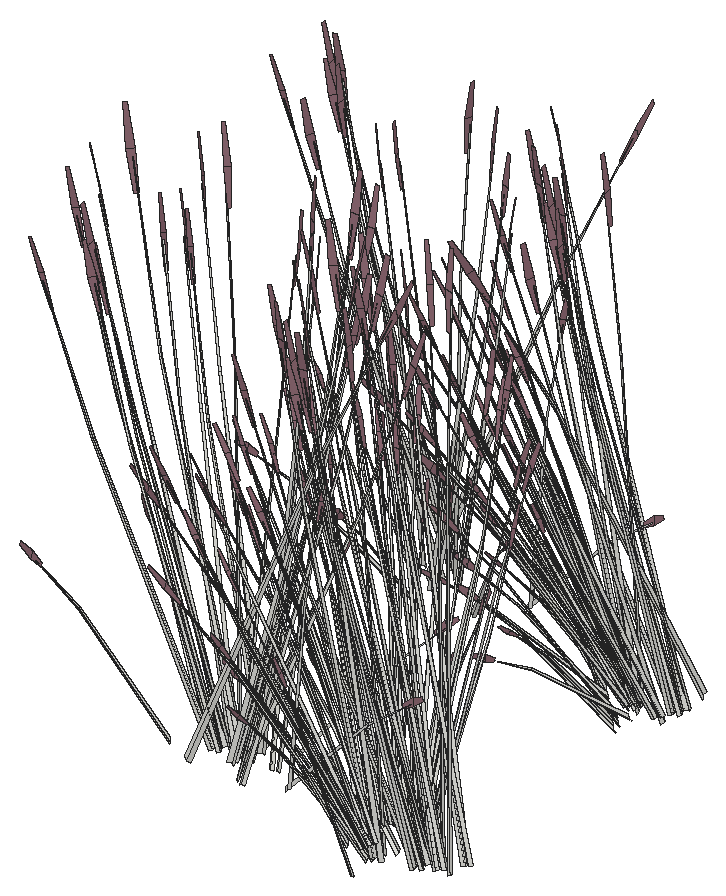
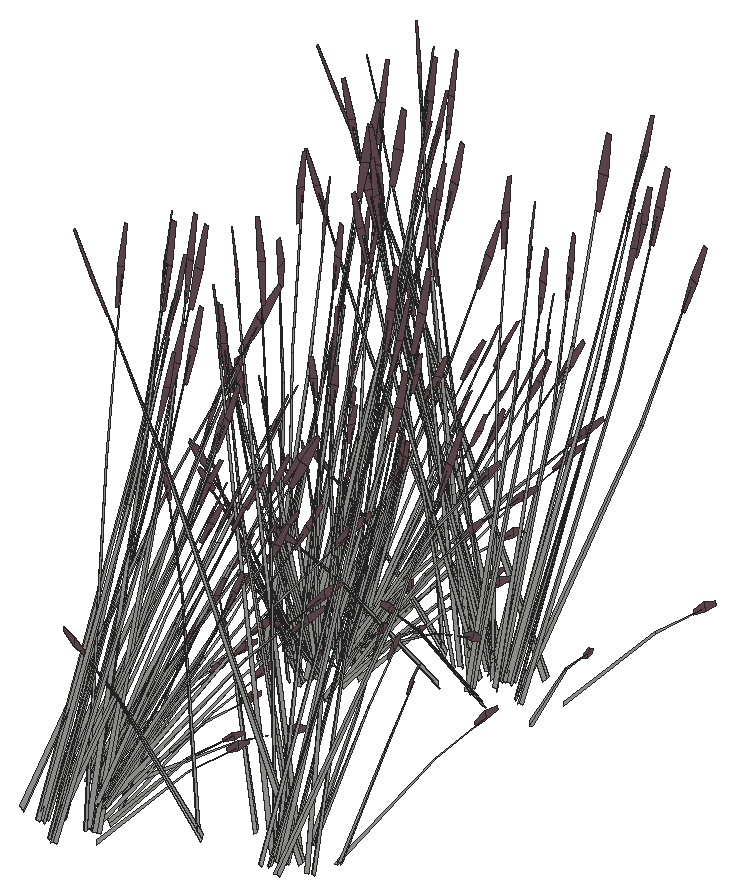
# SketchUp Ruby script. Lengths in inches.
U = 1.inch
M = Sketchup.active_model
def pt(a) = Geom::Point3d.new(a.map { |v| v * U })
def face(e, loops, mat)
  f = e.add_face(loops[0].map { |a| pt(a) })
  loops[1..].each { |l| e.add_face(l.map { |a| pt(a) }).erase! }
  f.material = f.back_material = mat if mat
  f
end
# faces: each face lists its corners as indices into pts; further lists are holes
def faces(e, pts, list, mat = nil) = list.each { |f| face(e, (f[0].is_a?(Array) ? f : [f]).map { |l| l.map { |i| pts[i] } }, mat) }
# xy, xz, yz: faces in a plane at the given z, y or x. An outline is a flat list of corners, or four numbers for a rectangle; further outlines are holes
def ring(l) = l.size == 4 ? [[l[0], l[1]], [l[2], l[1]], [l[2], l[3]], [l[0], l[3]]] : l.each_slice(2).to_a
def flat(e, list, mat, &to3) = list.each { |f| face(e, (f[0].is_a?(Array) ? f : [f]).map { |l| ring(l).map { |u, v| to3.(u, v) } }, mat) }
def xy(e, z, list, mat = nil) = flat(e, list, mat) { |x, y| [x, y, z] }
def xz(e, y, list, mat = nil) = flat(e, list, mat) { |x, z| [x, y, z] }
def yz(e, x, list, mat = nil) = flat(e, list, mat) { |y, z| [x, y, z] }
def lines(e, pts, list) = list.each { |a, b| e.add_line(pt(pts[a]), pt(pts[b])) }
# prism: a flat outline (further loops are holes) pulled along v
def prism(e, loops, v, mat = nil)
  f = face(e, loops, mat); d = Geom::Vector3d.new(v.map { |x| x * U })
  f.pushpull(f.normal.samedirection?(d) ? d.length : -d.length)
end
def box(e, o, s, mat = nil) = prism(e, [[o, [o[0] + s[0], o[1], o[2]], [o[0] + s[0], o[1] + s[1], o[2]], [o[0], o[1] + s[1], o[2]]]], [0, 0, s[2]], mat)
def at(x, y, z, deg = 0) = Geom::Transformation.translation(pt([x, y, z])) * Geom::Transformation.rotation(ORIGIN, Z_AXIS, deg.degrees)
def axes(o, x, y, z) = Geom::Transformation.new([*x, 0, *y, 0, *z, 0, *pt(o).to_a, 1])
def part(name) = M.definitions.add(name)
# library, detail: a bought-in or finely detailed component or shape, given as its bounding box
def library(name, o, s) = part(name).tap { |d| box(d.entities, o, s) }
def detail(e, o, s) = box(e.add_group.entities, o, s)
def put(e, d, t, mat = nil) = e.add_instance(d, t).tap { |i| i.material = mat if mat }
def group(e, t, mat = nil) = e.add_group.tap { |g| g.transformation = t; g.material = mat if mat }.entities
root = M.entities
M.materials.add("LightPink_Translucent").color = [144, 107, 117]
c1 = part("blade")
p = [[2.15,0.21,22],[0,0.17,0],[0.09,0.45,0],[2.18,0.31,22],[2.29,0.31,22],[0.38,0.45,0],
  [2.48,0.24,33],[2.49,0.24,33],[2.48,0.22,33]]
faces(c1.entities,p,[[0,1,2,3],[4,5,2,3],[6,3,4,7],[8,0,3,6]])
c2 = part("seeds")
p = [[0.3,-0.1,1.38],[-0.01,-0.03,1.59],[-0.01,-0.03,0.03],[0.14,-0.07,-0.07],[0.29,-0.03,3],[0.15,0.01,3.11]]
faces(c2.entities,p,[[0,1,2,3],[1,0,4,5]],"LightPink_Translucent")
c3 = part("blade with seeds")
put(c3.entities,c1,at(0,0,0))
put(c3.entities,c2,axes([2.4,0.25,30.99],[1.5799,-0.05474,1.17369],[-0.12525,1.92788,0.29478],[-0.07173,-0.02425,1.56792]))
put(root,c3,axes([47.72,595.87,44.06],[-1.27479,-0.1698,-0.62353],[0.26901,-1.04736,-0.16365],[-0.38043,-0.12691,1.37633]))
put(root,c3,axes([47.45,555.5625,43.49],[0.03108,0.16322,1.76342],[-0.62654,0.85237,-0.26939],[-0.44504,-0.04296,0.30037]))
put(root,c3,axes([45.54,590.14,43.49],[-0.11871,0.13643,1.76342],[-1.19964,0.29415,-0.26939],[-0.2898,-0.26759,0.30037]))
put(root,c3,axes([47.12,560.13,43.49],[0.16438,0.10347,1.76342],[0.27873,0.95868,-0.26939],[-0.36432,0.20444,0.30037]))
put(root,c3,axes([44.8,590.66,44.13],[-0.35352,0.84566,-0.03893],[-1.08806,-0.26014,-0.17649],[-0.1652,-0.13832,0.58215]))
put(root,c3,axes([51.55,557.04,44.06],[-1.27479,-0.1698,-0.62353],[0.26901,-1.04736,-0.16365],[-0.38043,-0.12691,1.37633]))
put(root,c3,axes([48.38,595.54,44.21],[-0.73619,-0.86927,-0.44739],[1.11511,-0.61213,0.21531],[-0.23824,-0.10756,1.43643]))
put(root,c3,axes([49.88,559.03,44.02],[-1.14694,-0.51783,-0.49651],[0.68554,-0.92854,0],[-0.26122,-0.11794,1.57504]))
put(root,c3,axes([48.49,596.03,44.4375],[0.32481,-1.2272,-0.23429],[1.54007,0.21392,0.51271],[-0.26911,-0.16947,1.5644]))
put(root,c3,axes([44.56,593.74,44.02],[0,-1.03566,-0.49651],[1.37109,0,0],[0,-0.23588,1.57504]))
put(root,c3,axes([48.14,594.9375,44.67],[-1.38012,-0.49416,-0.29095],[0.66454,-1.04299,-0.50002],[-0.04337,-0.25608,1.59708]))
put(root,c3,axes([53,557.2,44.67],[-1.23732,0.68758,-0.29095],[-0.8228,-0.97154,-0.50002],[-0.30528,-0.09867,1.59708]))
put(root,c3,axes([50.2,558.64,44.03],[-0.28787,-0.90242,-0.30978],[1.14332,-0.25625,0.30978],[-0.23049,-0.10406,1.38974]))
put(root,c3,axes([47.52,593.89,44.1],[-0.50328,-1.06202,-0.69835],[1.44974,-0.38248,-0.18329],[-0.05563,-0.35963,1.54149]))
put(root,c3,axes([53.82,557.95,44.06],[-0.82544,0.77843,-0.62353],[-1.0254,-0.70586,-0.16365],[-0.33076,0.19418,1.37633]))
put(root,c3,axes([45.15,593.76,44.03],[0.85545,-0.64616,-0.30978],[0.85545,0.64616,0.30978],[0,-0.20813,1.38974]))
put(root,c3,axes([49.01,589.58,44.13],[-0.84686,0.59414,-0.03893],[-0.77596,-0.65071,-0.17649],[-0.05463,-0.18438,0.58215]))
put(root,c3,axes([54.39,557.51,44.46],[-1.19666,-0.83357,-0.25192],[1.00694,-0.93603,0.5513],[-0.32224,0.09751,1.68216]))
put(root,c3,axes([52.21,556.71,44.21],[-0.73619,-0.86927,-0.44739],[1.11511,-0.61213,0.21531],[-0.23824,-0.10756,1.43643]))
put(root,c3,axes([53.78,557.33,44.21],[-1.33077,0.06393,-0.44739],[-0.12035,-1.06125,0.21531],[-0.23824,0.10756,1.43643]))
put(root,c3,axes([52.32,557.21,44.4375],[0.32481,-1.2272,-0.23429],[1.54007,0.21392,0.51271],[-0.26911,-0.16947,1.5644]))
put(root,c3,axes([55.18,560.07,44.02],[-1.14694,0.51783,-0.49651],[-0.68554,-0.92854,0],[-0.26122,0.11794,1.57504]))
put(root,c3,axes([49.22,588.86,43.49],[-0.20555,0.03731,1.76342],[-1.13672,-0.42002,-0.26939],[0.01907,-0.35034,0.30037]))
put(root,c3,axes([54.91,559.66,44.03],[-1.14332,-0.25625,-0.30978],[0.28787,-0.90242,0.30978],[-0.23049,0.10406,1.38974]))
put(root,c3,axes([48.29,594.16,44.21],[0.59459,-0.93321,-0.44739],[1.23546,0.44912,0.21531],[0,-0.21512,1.43643]))
put(root,c3,axes([54.71,557.05,44.67],[0.1428,1.18174,-0.29095],[-1.48733,0.07145,-0.50002],[-0.26191,0.15741,1.59708]))
put(root,c3,axes([52.19,560.23,43.49],[0.19833,-0.05635,1.76342],[1.19302,0.31018,-0.26939],[0.03489,0.3496,0.30037]))
put(root,c3,axes([48.83,593.7,44.67],[-0.1428,-1.18174,-0.29095],[1.48733,-0.07145,-0.50002],[0.26191,-0.15741,1.59708]))
put(root,c3,axes([55.26,556.58,44.21],[-0.59459,0.93321,-0.44739],[-1.23546,-0.44912,0.21531],[0,0.21512,1.43643]))
put(root,c3,axes([48.64,591.08,44.03],[1.14332,0.25625,-0.30978],[-0.28787,0.90242,0.30978],[0.23049,-0.10406,1.38974]))
put(root,c3,axes([48.37,590.67,44.02],[1.14694,-0.51783,-0.49651],[0.68554,0.92854,0],[0.26122,-0.11794,1.57504]))
put(root,c3,axes([58.4,556.98,44.03],[-0.85545,0.64616,-0.30978],[-0.85545,-0.64616,0.30978],[0,0.20813,1.38974]))
put(root,c3,axes([49.73,592.8,44.06],[0.82544,-0.77843,-0.62353],[1.0254,0.70586,-0.16365],[0.33076,-0.19418,1.37633]))
put(root,c3,axes([55.96,556.87,44.09],[0.44936,0.94823,-0.69212],[-1.29441,0.3415,-0.18165],[0.04967,0.32109,1.52773]))
put(root,c3,axes([69.75,555.49,41.15],[0.50831,-0.02346,1.71376],[-0.33721,1.01661,0.13857],[-0.72439,-0.06288,0.73262]))
put(root,c3,axes([69.75,591.94,40.8125],[0.50831,-0.02346,1.71376],[-0.33721,1.01661,0.13857],[-0.72439,-0.06288,0.73262]))
put(root,c3,axes([55.4,555.81,44.67],[1.38012,0.49416,-0.29095],[-0.66454,1.04299,-0.50002],[0.04337,0.25608,1.59708]))
put(root,c3,axes([69.96,557.28,41.15],[0.42521,-0.21906,1.71376],[0.35798,1.01226,0.13857],[-0.66754,0.22878,0.73262]))
put(root,c3,axes([58.99,557.01,44.02],[0,1.03566,-0.49651],[-1.37109,0,0],[0,0.23588,1.57504]))
put(root,c3,axes([68.64,559,39.87],[0.42589,0.08502,1.43002],[0.2745,0.86839,-0.30754],[-0.57851,0.16255,0.61141]))
put(root,c3,axes([47.43,592.93,43.59],[-1.20625,0.41464,1.28929],[-0.38394,-1.1897,0.50096],[0.74071,0.01979,1.46642]))
put(root,c3,axes([72.41,556.22,40.62],[0.34834,-0.14982,1.77064],[0.12012,1.04605,0.13857],[-0.75452,0.1388,0.63284]))
put(root,c3,axes([54.25,590.64,43.49],[-0.18342,-0.08159,1.76342],[-0.47115,-0.9115,-0.26939],[0.31784,-0.24736,0.30037]))
put(root,c3,axes([55.14,558.22,44.18],[1.2866,-0.3514,-0.19198],[0.45209,1.01223,0.00008],[0.14202,-0.03884,1.73897]))
put(root,c3,axes([68.66,556.92,41.99],[-0.20012,0.13446,1.74944],[0.01702,0.98243,-0.27667],[-0.45871,0.12776,0.14031]))
put(root,c3,axes([71.27,554.54,42.26],[-1.22504,-0.02494,-0.71045],[0.08228,-1.05005,0.08574],[-0.51899,-0.11081,1.00501]))
put(root,c3,axes([71.27,590.99,41.92],[-1.22504,-0.02494,-0.71045],[0.08228,-1.05005,0.08574],[-0.51899,-0.11081,1.00501]))
put(root,c3,axes([70.29,554.8,39.87],[0.23927,0.28834,1.43002],[-0.55135,0.78376,-0.30754],[-0.56612,-0.18733,0.61141]))
put(root,c3,axes([70.29,591.25,39.53],[0.23927,0.28834,1.43002],[-0.55135,0.78376,-0.30754],[-0.56612,-0.18733,0.61141]))
put(root,c3,axes([55.16,555.21,44.21],[0.73619,0.86927,-0.44739],[-1.11511,0.61213,0.21531],[0.23824,0.10756,1.43643]))
put(root,c3,axes([69.31,556.36,41.8],[-1.01846,-0.28891,-0.35414],[0.29705,-0.84289,0.4572],[-0.41005,0.07729,0.87481]))
put(root,c3,axes([69.31,592.81,41.46],[-1.01846,-0.28891,-0.35414],[0.29705,-0.84289,0.4572],[-0.41005,0.07729,0.87481]))
put(root,c3,axes([70.71,590.3,40.8125],[0.45521,0.17844,1.71376],[-0.94204,0.74856,0.13857],[-0.58713,-0.33769,0.73262]))
put(root,c3,axes([57.42,594.32,44.26],[-0.75977,-0.66224,-0.06488],[0.83212,-0.6068,-0.29416],[0.23578,-0.04272,0.97024]))
put(root,c3,axes([66.4375,557.91,41.99],[0.1564,0.02778,1.77383],[0.48382,0.91506,-0.16761],[-0.32016,0.24017,0.31391]))
put(root,c3,axes([70,556.79,41.96],[-0.332,0.94205,-0.51099],[-1.13828,-0.3229,-0.3958],[-0.45829,0.08638,0.97773]))
put(root,c3,axes([70.87,554.75,41.96],[-0.88986,0.68603,-0.51099],[-0.77932,-0.72471,-0.3958],[-0.45212,-0.10438,0.97773]))
put(root,c3,axes([70.87,591.2,41.62],[-0.88986,0.68603,-0.51099],[-0.77932,-0.72471,-0.3958],[-0.45212,-0.10438,0.97773]))
put(root,c3,axes([69.43,556.73,38.77],[0.03108,0.16322,1.76342],[-0.62654,0.85237,-0.26939],[-0.44504,-0.04296,0.30037]))
put(root,c3,axes([69.43,593.18,38.43],[0.03108,0.16322,1.76342],[-0.62654,0.85237,-0.26939],[-0.44504,-0.04296,0.30037]))
put(root,c3,axes([57.18,553.28,44.03],[0.28787,0.90242,-0.30978],[-1.14332,0.25625,0.30978],[0.23049,0.10406,1.38974]))
put(root,c3,axes([69.61,552.83,41.99],[0.09085,0.10335,1.77383],[-0.43798,0.92907,-0.16761],[-0.44357,0.00672,0.31391]))
put(root,c3,axes([69.61,589.28,41.64],[0.09085,0.10335,1.77383],[-0.43798,0.92907,-0.16761],[-0.44357,0.00672,0.31391]))
put(root,c3,axes([67.75,560.82,40.04],[0.51072,-0.46938,1.1486],[0.20153,0.74307,0.84392],[-0.36908,0.13305,0.25299]))
put(root,c3,axes([54.38,554.72,44.67],[1.23732,-0.68758,-0.29095],[0.8228,0.97154,-0.50002],[0.30528,0.09867,1.59708]))
put(root,c3,axes([70.625,588.66,41.65],[-0.26368,-0.00731,1.74944],[-0.83946,0.73103,-0.27667],[-0.44791,-0.14937,0.14031]))
put(root,c3,axes([69.54,556.26,42.01],[0.34623,-0.9443,0.48003],[1.13828,0.3229,0.3958],[-0.44763,0.05675,0.9933]))
put(root,c3,axes([69.54,592.7,41.67],[0.34623,-0.9443,0.48003],[1.13828,0.3229,0.3958],[-0.44763,0.05675,0.9933]))
put(root,c3,axes([69.95,555.98,42.3125],[0.6166,0.93779,-0.1216],[-1.09436,0.46085,-0.67495],[-0.46117,0.12373,1.02557]))
put(root,c3,axes([71.33,554.04,42.3125],[-0.06562,1.05324,-0.1216],[-1.2424,-0.02879,-0.67495],[-0.4785,-0.07316,1.02557]))
put(root,c3,axes([71.33,590.48,41.97],[-0.06562,1.05324,-0.1216],[-1.2424,-0.02879,-0.67495],[-0.4785,-0.07316,1.02557]))
put(root,c3,axes([70.54,554.11,41.8],[-0.69728,-0.64842,-0.35414],[0.79619,-0.61382,0.4572],[-0.40453,-0.09339,0.87481]))
put(root,c3,axes([70.54,590.56,41.46],[-0.69728,-0.64842,-0.35414],[0.79619,-0.61382,0.4572],[-0.40453,-0.09339,0.87481]))
put(root,c3,axes([69.46,556,42.01],[-0.4501,-0.70615,0.0643],[0.82077,-0.34564,0.50621],[-0.36181,0.0682,0.77189]))
put(root,c3,axes([69.46,592.45,41.67],[-0.4501,-0.70615,0.0643],[0.82077,-0.34564,0.50621],[-0.36181,0.0682,0.77189]))
put(root,c3,axes([71.52,557.96,41.15],[0.30609,-0.31822,1.71376],[0.77286,0.85893,0.13857],[-0.53009,0.39116,0.73262]))
put(root,c3,axes([69.68,558.79,41.8],[-1.06674,0.14801,-0.35414],[-0.28168,-0.84611,0.4572],[-0.30569,0.22726,0.87481]))
put(root,c3,axes([69.1,561.3,38.77],[0.16438,0.10347,1.76342],[0.27873,0.95868,-0.26939],[-0.36432,0.20444,0.30037]))
put(root,c3,axes([51.26,554.11,43.59],[-1.20625,0.41464,1.28929],[-0.38394,-1.1897,0.50096],[0.74071,0.01979,1.46642]))
put(root,c3,axes([68.86,555.66,40.04],[0.78239,-0.07411,1.1486],[-0.49629,0.65296,0.84392],[-0.38663,-0.09795,0.25299]))
put(root,c3,axes([68.86,592.11,39.7],[0.78239,-0.07411,1.1486],[-0.49629,0.65296,0.84392],[-0.38663,-0.09795,0.25299]))
put(root,c3,axes([69.82,558.61,42.01],[-0.30393,-0.95317,0.48003],[1.19224,-0.16542,0.3958],[-0.35138,0.22417,0.9933]))
put(root,c3,axes([70.43,590.3125,42.03],[1.01205,-0.7643,0.53763],[0.87284,0.81167,0.4433],[-0.47482,-0.14098,1.11249]))
put(root,c3,axes([69.58,558.42,42.01],[-0.8413,-0.43556,0.0643],[0.48981,-0.62025,0.50621],[-0.26973,0.20053,0.77189]))
put(root,c3,axes([57.5,552.89,44.02],[1.14694,0.51783,-0.49651],[-0.68554,0.92854,0],[0.26122,0.11794,1.57504]))
put(root,c3,axes([57.44,560.26,43.49],[0.08928,-0.14952,1.76342],[1.12407,-0.44035,-0.26939],[0.34078,0.22791,0.30037]))
put(root,c3,axes([71.29,558.74,41.15],[0.22818,-0.35597,1.71376],[0.95725,0.73667,0.13857],[-0.43183,0.45914,0.73262]))
put(root,c3,axes([70.38,556.27,42.33],[1.01846,0.28891,0.35414],[-0.29705,0.84289,-0.4572],[-0.41005,0.07729,0.87481]))
put(root,c3,axes([55.83,554.875,44.06],[1.27479,0.1698,-0.62353],[-0.26901,1.04736,-0.16365],[0.38043,0.12691,1.37633]))
put(root,c3,axes([70.56,558.89,41.96],[0.31482,0.94565,-0.51099],[-1.19224,0.16542,-0.3958],[-0.34166,0.254,0.97773]))
put(root,c3,axes([61.25,555.49,44.26],[-0.75977,-0.66224,-0.06488],[0.83212,-0.6068,-0.29416],[0.23578,-0.04272,0.97024]))
put(root,c3,axes([70.89,553.86,42.01],[0.06171,-0.78753,0.0643],[0.9318,0.02159,0.50621],[-0.35694,-0.08241,0.77189]))
put(root,c3,axes([70.89,590.31,41.67],[0.06171,-0.78753,0.0643],[0.9318,0.02159,0.50621],[-0.35694,-0.08241,0.77189]))
put(root,c3,axes([68.7,560.59,41.99],[-0.03046,0.20495,1.74944],[0.86449,0.71297,-0.27667],[-0.22632,0.33716,0.14031]))
put(root,c3,axes([73.53,558.21,39.34],[-1.27479,-0.1698,-0.62353],[0.26901,-1.04736,-0.16365],[-0.38043,-0.12691,1.37633]))
put(root,c3,axes([73.53,594.66,38.99],[-1.27479,-0.1698,-0.62353],[0.26901,-1.04736,-0.16365],[-0.38043,-0.12691,1.37633]))
put(root,c3,axes([73.76,588.95,42.37],[-0.81789,0.99285,-0.13619],[-1.18445,-0.572,-0.75594],[-0.41173,-0.28051,1.14864]))
put(root,c3,axes([56.85,594.55,43.49],[-0.06405,-0.15723,1.76342],[0.44421,-0.91974,-0.26939],[0.4481,-0.01323,0.30037]))
put(root,c3,axes([71.53,554.45,42.33],[0.69728,0.64842,0.35414],[-0.79619,0.61382,-0.4572],[-0.40453,-0.09339,0.87481]))
put(root,c3,axes([71.53,590.9,41.99],[0.69728,0.64842,0.35414],[-0.79619,0.61382,-0.4572],[-0.40453,-0.09339,0.87481]))
put(root,c3,axes([73.4,589.75,41.92],[-1.04497,-0.50058,-0.71045],[0.74264,-0.8772,0.08574],[-0.3786,-0.29889,1.00501]))
put(root,c3,axes([72.91,589.78,41.62],[-1.20928,0.24619,-0.51099],[-0.21154,-0.93233,-0.3958],[-0.32481,-0.26718,0.97773]))
put(root,c3,axes([71.86,560.19,39.3],[-1.14694,-0.51783,-0.49651],[0.68554,-0.92854,0],[-0.26122,-0.11794,1.57504]))
put(root,c3,axes([71.86,596.64,38.95],[-1.14694,-0.51783,-0.49651],[0.68554,-0.92854,0],[-0.26122,-0.11794,1.57504]))
put(root,c3,axes([71.35,588.93,38.43],[-0.11871,0.13643,1.76342],[-1.19964,0.29415,-0.26939],[-0.2898,-0.26759,0.30037]))
put(root,c3,axes([70,558.21,42.3125],[1.1336,0.57106,-0.1216],[-0.65308,0.827,-0.67495],[-0.32027,0.28747,1.02557]))
put(root,c3,axes([72.56,560.82,39.65],[-0.7662,1.03778,0],[-1.28187,-0.57875,-0.51607],[-0.29196,-0.13181,1.63711]))
put(root,c3,axes([68.125,560.69,42.92],[1.08141,0.27645,-0.06488],[-0.33265,0.85086,-0.29416],[-0.17688,0.12919,0.97024]))
put(root,c3,axes([70.55,558.29,42.33],[1.06674,-0.14801,0.35414],[0.28168,0.84611,-0.4572],[-0.30569,0.22726,0.87481]))
put(root,c3,axes([71.16,562.32,39.87],[0.38672,-0.16338,1.43002],[0.95481,0.49262,-0.30754],[-0.28419,0.42626,0.61141]))
put(root,c3,axes([70.61,553,39.41],[-0.35352,0.84566,-0.03893],[-1.08806,-0.26014,-0.17649],[-0.1652,-0.13832,0.58215]))
put(root,c3,axes([70.61,589.45,39.0625],[-0.35352,0.84566,-0.03893],[-1.08806,-0.26014,-0.17649],[-0.1652,-0.13832,0.58215]))
put(root,c3,axes([73.44,586.59,41.64],[-0.02286,0.12414,1.77383],[-1.12758,0.45052,-0.16761],[-0.33182,-0.23029,0.31391]))
put(root,c3,axes([72.23,588.39,39.53],[-0.07421,0.33879,1.43002],[-1.08488,0.28361,-0.30754],[-0.25359,-0.4379,0.61141]))
put(root,c3,axes([72.59,589.27,40.8125],[0.28013,0.33252,1.71376],[-1.29445,0.27994,0.13857],[-0.29256,-0.52202,0.73262]))
put(root,c3,axes([74.98,558.37,39.94],[-1.23732,0.68758,-0.29095],[-0.8228,-0.97154,-0.50002],[-0.30528,-0.09867,1.59708]))
put(root,c3,axes([74.98,594.8125,39.6],[-1.23732,0.68758,-0.29095],[-0.8228,-0.97154,-0.50002],[-0.30528,-0.09867,1.59708]))
put(root,c3,axes([71.56,560.54,42.01],[-0.87265,-0.70663,0.48003],[0.92674,-0.60943,0.3958],[-0.16097,0.33153,0.9933]))
put(root,c3,axes([73.04,589.09,41.46],[-0.18927,-0.83419,-0.35414],[1.08199,-0.22027,0.4572],[-0.29062,-0.23905,0.87481]))
put(root,c3,axes([70.02,556.87,39.65],[-1.53239,0,0],[0,-1.1575,-0.51607],[0,-0.26363,1.63711]))
put(root,c3,axes([70.02,593.31,39.31],[-1.53239,0,0],[0,-1.1575,-0.51607],[0,-0.26363,1.63711]))
put(root,c3,axes([72.18,559.81,39.31],[-0.28787,-0.90242,-0.30978],[1.14332,-0.25625,0.30978],[-0.23049,-0.10406,1.38974]))
put(root,c3,axes([72.18,596.26,38.96],[-0.28787,-0.90242,-0.30978],[1.14332,-0.25625,0.30978],[-0.23049,-0.10406,1.38974]))
put(root,c3,axes([71.24,560.47,42.01],[-1.00708,-0.04826,0.0643],[0.02761,-0.72867,0.50621],[-0.10538,0.27912,0.77189]))
put(root,c3,axes([71.55,560.75,41.8],[-0.82919,0.54528,-0.35414],[-0.78493,-0.62262,0.4572],[-0.11943,0.31634,0.87481]))
put(root,c3,axes([75.8,559.12,39.34],[-0.82544,0.77843,-0.62353],[-1.0254,-0.70586,-0.16365],[-0.33076,0.19418,1.37633]))
put(root,c3,axes([73.68,589.77,41.99],[0.18927,0.83419,0.35414],[-1.08199,0.22027,-0.4572],[-0.29062,-0.23905,0.87481]))
put(root,c3,axes([68.6,562.6875,41.99],[0.13903,-0.06253,1.77383],[1.14912,0.41591,-0.16761],[-0.027,0.34629,0.31391]))
put(root,c3,axes([71.21,556.5625,39.61],[-1.1399,0.87071,0.30756],[-1.1406,-0.86155,-0.36492],[-0.03981,-0.24727,1.64885]))
put(root,c3,axes([71.21,593.01,39.27],[-1.1399,0.87071,0.30756],[-1.1406,-0.86155,-0.36492],[-0.03981,-0.24727,1.64885]))
put(root,c3,axes([60.68,555.72,43.49],[-0.06405,-0.15723,1.76342],[0.44421,-0.91974,-0.26939],[0.4481,-0.01323,0.30037]))
put(root,c3,axes([75.9,595.42,40.26],[1.05902,0.41762,1.51261],[-1.03748,0.89969,0.59816],[-0.46471,-0.53324,1.26806]))
put(root,c3,axes([71.86,587.84,39.7],[0.63926,0.36046,1.1486],[-0.93099,0.21668,0.84392],[-0.1992,-0.27702,0.25299]))
put(root,c3,axes([76.37,558.68,39.74],[-1.19666,-0.83357,-0.25192],[1.00694,-0.93603,0.5513],[-0.32224,0.09751,1.68216]))
put(root,c3,axes([74.19,557.88,39.49],[-0.73619,-0.86927,-0.44739],[1.11511,-0.61213,0.21531],[-0.23824,-0.10756,1.43643]))
put(root,c3,axes([74.19,594.33,39.15],[-0.73619,-0.86927,-0.44739],[1.11511,-0.61213,0.21531],[-0.23824,-0.10756,1.43643]))
put(root,c3,axes([72.11,560.17,42.62],[-0.03189,0.95798,-0.7886],[-1.34277,-0.06434,0.09517],[-0.14171,0.40585,1.11556]))
put(root,c3,axes([72.08,562.87,40.04],[-0.03171,-0.6158,1.1486],[0.7925,0.43922,0.84392],[-0.15586,0.29352,0.25299]))
put(root,c3,axes([73.2,588.79,42.03],[1.36515,-0.26619,0.53763],[0.23692,1.04421,0.4433],[-0.32106,-0.30775,1.11249]))
put(root,c3,axes([75.76,558.5,39.49],[-1.33077,0.06393,-0.44739],[-0.12035,-1.06125,0.21531],[-0.23824,0.10756,1.43643]))
put(root,c3,axes([73.51,589.01,41.67],[0.55698,-0.6579,0.0643],[0.79316,0.38303,0.50621],[-0.25643,-0.21093,0.77189]))
put(root,c3,axes([73.22,560.28,39.76],[1.14694,0.51783,0.49651],[-0.68554,0.92854,0],[-0.26122,-0.11794,1.57504]))
put(root,c3,axes([71.66,561.52,40.64],[0.02693,-0.53464,1.54345],[1.21102,0.2824,0.21329],[-0.10493,0.5698,0.72882]))
put(root,c3,axes([74.3,558.375,39.72],[0.32481,-1.2272,-0.23429],[1.54007,0.21392,0.51271],[-0.26911,-0.16947,1.5644]))
put(root,c3,axes([74.3,594.83,39.375],[0.32481,-1.2272,-0.23429],[1.54007,0.21392,0.51271],[-0.26911,-0.16947,1.5644]))
put(root,c3,axes([74.86,558.67,39.89],[-0.23642,0.92427,0.1448],[-1.15506,-0.16044,-0.41347],[-0.21021,-0.09491,1.26744]))
put(root,c3,axes([74.73,587.0625,41.65],[-0.18744,-0.14521,1.74944],[-1.25089,0.09206,-0.27667],[-0.19964,-0.34731,0.14031]))
put(root,c3,axes([77.16,561.24,39.3],[-1.14694,0.51783,-0.49651],[-0.68554,-0.92854,0],[-0.26122,0.11794,1.57504]))
put(root,c3,axes([70.37,592.53,38.95],[0,-1.03566,-0.49651],[1.37109,0,0],[0,-0.23588,1.57504]))
put(root,c3,axes([70.95,557.04,39.76],[0,1.03566,0.49651],[-1.37109,0,0],[0,-0.23588,1.57504]))
put(root,c3,axes([70.95,593.49,39.41],[0,1.03566,0.49651],[-1.37109,0,0],[0,-0.23588,1.57504]))
put(root,c3,axes([77.23,560.96,39.47],[-0.75665,-1.04141,-0.05142],[1.28187,-0.57875,0.51607],[-0.31588,0.09915,1.6363]))
put(root,c3,axes([72.38,560.49,42.28],[0.87728,0.69587,-0.5672],[-0.92674,0.60943,-0.43934],[-0.13348,0.35356,1.08528]))
put(root,c3,axes([76.89,560.83,39.31],[-1.14332,-0.25625,-0.30978],[0.28787,-0.90242,0.30978],[-0.23049,0.10406,1.38974]))
put(root,c3,axes([71.99,559.98,42.33],[0.82919,-0.54528,0.35414],[0.78493,0.62262,-0.4572],[-0.11943,0.31634,0.87481]))
put(root,c3,axes([73.95,557.28,39.94],[-1.38012,-0.49416,-0.29095],[0.66454,-1.04299,-0.50002],[-0.04337,-0.25608,1.59708]))
put(root,c3,axes([73.95,593.73,39.6],[-1.38012,-0.49416,-0.29095],[0.66454,-1.04299,-0.50002],[-0.04337,-0.25608,1.59708]))
put(root,c3,axes([77.55,556.97,40.12],[-0.03348,-0.97511,1.41272],[1.51511,0.25277,0.59816],[-0.35835,0.53357,1.3335]))
put(root,c3,axes([71.46,560.125,42.68],[1.34686,0.05131,-0.13498],[-0.03681,0.97156,-0.74919],[-0.09356,0.37418,1.13838]))
put(root,c3,axes([71.43,561.54,40.1],[1.11329,-0.1834,0.06507],[0.25594,0.73887,-0.86304],[-0.07058,0.37403,0.7736]))
put(root,c3,axes([76.69,558.21,39.94],[0.1428,1.18174,-0.29095],[-1.48733,0.07145,-0.50002],[-0.26191,0.15741,1.59708]))
put(root,c3,axes([73.33,592.68,39.03],[-0.50328,-1.06202,-0.69835],[1.44974,-0.38248,-0.18329],[-0.05563,-0.35963,1.54149]))
put(root,c3,axes([76.63,589.3,41.97],[-1.19922,0.48218,-0.1216],[-0.58932,-0.85579,-0.67495],[-0.15822,-0.36063,1.02557]))
put(root,c3,axes([75.6,589.35,41.62],[-1.20468,-0.25962,-0.51099],[0.41292,-0.89013,-0.3958],[-0.11046,-0.35838,0.97773]))
put(root,c3,axes([73.38,559.49,41.15],[-0.02999,-0.3975,1.71376],[1.30002,0.26369,0.13857],[-0.08041,0.56647,0.73262]))
